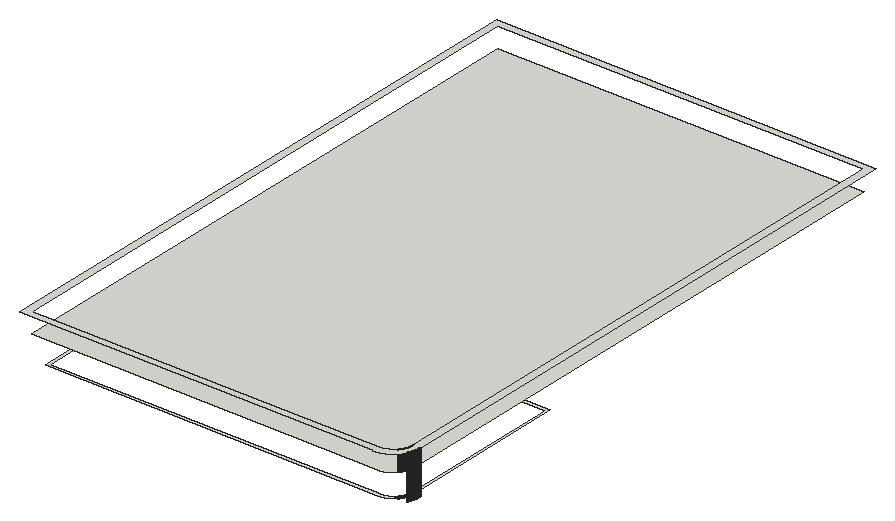
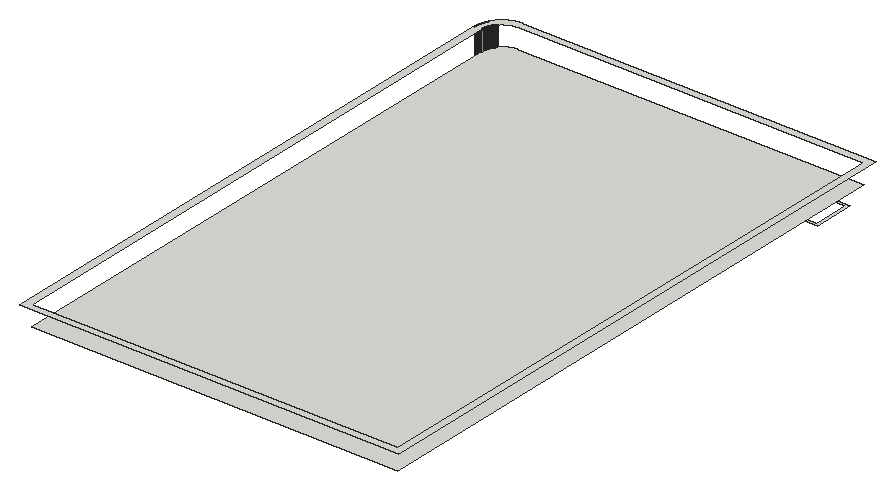
# SketchUp Ruby script. Lengths in inches.
U = 1.inch
M = Sketchup.active_model
def pt(a) = Geom::Point3d.new(a.map { |v| v * U })
def face(e, loops, mat)
  f = e.add_face(loops[0].map { |a| pt(a) })
  loops[1..].each { |l| e.add_face(l.map { |a| pt(a) }).erase! }
  f.material = f.back_material = mat if mat
  f
end
# faces: each face lists its corners as indices into pts; further lists are holes
def faces(e, pts, list, mat = nil) = list.each { |f| face(e, (f[0].is_a?(Array) ? f : [f]).map { |l| l.map { |i| pts[i] } }, mat) }
# xy, xz, yz: faces in a plane at the given z, y or x. An outline is a flat list of corners, or four numbers for a rectangle; further outlines are holes
def ring(l) = l.size == 4 ? [[l[0], l[1]], [l[2], l[1]], [l[2], l[3]], [l[0], l[3]]] : l.each_slice(2).to_a
def flat(e, list, mat, &to3) = list.each { |f| face(e, (f[0].is_a?(Array) ? f : [f]).map { |l| ring(l).map { |u, v| to3.(u, v) } }, mat) }
def xy(e, z, list, mat = nil) = flat(e, list, mat) { |x, y| [x, y, z] }
def xz(e, y, list, mat = nil) = flat(e, list, mat) { |x, z| [x, y, z] }
def yz(e, x, list, mat = nil) = flat(e, list, mat) { |y, z| [x, y, z] }
def lines(e, pts, list) = list.each { |a, b| e.add_line(pt(pts[a]), pt(pts[b])) }
# prism: a flat outline (further loops are holes) pulled along v
def prism(e, loops, v, mat = nil)
  f = face(e, loops, mat); d = Geom::Vector3d.new(v.map { |x| x * U })
  f.pushpull(f.normal.samedirection?(d) ? d.length : -d.length)
end
def box(e, o, s, mat = nil) = prism(e, [[o, [o[0] + s[0], o[1], o[2]], [o[0] + s[0], o[1] + s[1], o[2]], [o[0], o[1] + s[1], o[2]]]], [0, 0, s[2]], mat)
def at(x, y, z, deg = 0) = Geom::Transformation.translation(pt([x, y, z])) * Geom::Transformation.rotation(ORIGIN, Z_AXIS, deg.degrees)
def axes(o, x, y, z) = Geom::Transformation.new([*x, 0, *y, 0, *z, 0, *pt(o).to_a, 1])
def part(name) = M.definitions.add(name)
# library, detail: a bought-in or finely detailed component or shape, given as its bounding box
def library(name, o, s) = part(name).tap { |d| box(d.entities, o, s) }
def detail(e, o, s) = box(e.add_group.entities, o, s)
def put(e, d, t, mat = nil) = e.add_instance(d, t).tap { |i| i.material = mat if mat }
def group(e, t, mat = nil) = e.add_group.tap { |g| g.transformation = t; g.material = mat if mat }.entities
root = M.entities
xy(root,231.5,[[[30,170,30,206,177,206,177,338,342,338,342,187.76,341.99,187.53,341.99,187.29,341.98,187.06,341.96,186.82,341.94,186.59,341.92,186.35,341.9,186.12,341.875,185.88,341.85,185.65,341.8125,185.42,341.78,185.18,341.7,184.72,341.65,184.49,341.61,184.26,341.56,184.03,341.5,183.8,341.45,183.57,341.39,183.34,341.32,183.11,341.26,182.89,341.19,182.66,341.12,182.4375,341.04,182.21,340.97,181.99,340.89,181.77,340.8,181.55,340.72,181.33,340.54,180.89,340.44,180.68,340.35,180.46,340.25,180.25,340.14,180.04,340.04,179.83,339.82,179.41,339.7,179.2,339.59,179,339.35,178.6,339.22,178.39,339.1,178.2,338.97,178,338.83,177.8,338.7,177.61,338.5625,177.42,338.42,177.23,338.28,177.04,338.14,176.86,337.99,176.67,337.84,176.49,337.6875,176.31,337.53,176.13,337.375,175.96,337.22,175.78,337.06,175.61,336.89,175.44,336.73,175.27,336.56,175.11,336.39,174.94,336.22,174.78,336.04,174.625,335.87,174.47,335.69,174.3125,335.51,174.16,335.33,174.01,335.14,173.86,334.96,173.72,334.77,173.58,334.58,173.4375,334.39,173.3,334.2,173.17,334,173.03,333.8,172.9,333.61,172.78,333.4,172.65,333,172.41,332.8,172.3,332.59,172.18,332.17,171.96,331.96,171.86,331.75,171.75,331.54,171.65,331.32,171.56,331.11,171.46,330.67,171.28,330.45,171.2,330.23,171.11,330.01,171.03,329.79,170.96,329.5625,170.88,329.34,170.81,329.11,170.74,328.89,170.68,328.66,170.61,328.43,170.55,328.2,170.5,327.97,170.44,327.74,170.39,327.51,170.35,327.28,170.3,326.82,170.22,326.58,170.1875,326.35,170.15,326.12,170.125,325.88,170.1,325.65,170.08,325.41,170.06,325.18,170.04,324.94,170.02,324.71,170.01,324.47,170.01,324.24,170],[32,172,324.21,172,324.42,172.01,324.63,172.01,325.05,172.03,325.26,172.05,325.46,172.07,325.88,172.11,326.3,172.17,326.5,172.2,326.71,172.23,326.92,172.27,327.12,172.31,327.33,172.35,327.53,172.39,327.74,172.44,327.9375,172.49,328.14,172.55,328.34,172.6,328.94,172.78,329.54,172.99,329.73,173.0625,329.93,173.14,330.12,173.22,330.32,173.3,330.51,173.38,331.08,173.65,331.26,173.74,331.45,173.84,331.63,173.9375,331.82,174.04,332,174.14,332.54,174.47,332.71,174.58,332.89,174.7,333.0625,174.8125,333.23,174.93,333.4,175.06,333.57,175.18,333.74,175.31,333.91,175.43,334.07,175.57,334.39,175.83,334.71,176.11,335.01,176.39,335.16,176.54,335.3125,176.6875,335.46,176.84,335.61,176.99,335.89,177.29,336.17,177.61,336.43,177.93,336.57,178.09,336.69,178.26,336.82,178.43,336.94,178.6,337.07,178.77,337.1875,178.9375,337.3,179.11,337.42,179.29,337.53,179.46,337.86,180,337.96,180.18,338.0625,180.37,338.16,180.55,338.26,180.74,338.35,180.92,338.62,181.49,338.7,181.68,338.78,181.88,338.86,182.07,338.9375,182.27,339.01,182.46,339.22,183.06,339.4,183.66,339.45,183.86,339.51,184.0625,339.56,184.26,339.61,184.47,339.65,184.67,339.69,184.88,339.73,185.08,339.77,185.29,339.8,185.5,339.83,185.7,339.89,186.12,339.93,186.54,339.95,186.74,339.97,186.95,339.99,187.37,339.99,187.58,340,187.79,340,336,179,336,179,204,32,204]]])
xy(root,252,[[18,170,324.24,170,324.47,170.01,324.71,170.01,324.94,170.02,325.18,170.04,325.41,170.06,325.65,170.08,325.88,170.1,326.12,170.125,326.35,170.15,326.58,170.1875,326.82,170.22,327.28,170.3,327.51,170.35,327.74,170.39,327.97,170.44,328.2,170.5,328.43,170.55,328.66,170.61,328.89,170.68,329.11,170.74,329.34,170.81,329.5625,170.88,329.79,170.96,330.01,171.03,330.23,171.11,330.45,171.2,330.67,171.28,331.11,171.46,331.32,171.56,331.54,171.65,331.75,171.75,331.96,171.86,332.17,171.96,332.59,172.18,332.8,172.3,333,172.41,333.4,172.65,333.61,172.78,333.8,172.9,334,173.03,334.2,173.17,334.39,173.3,334.58,173.4375,334.77,173.58,334.96,173.72,335.14,173.86,335.33,174.01,335.51,174.16,335.69,174.3125,335.87,174.47,336.04,174.625,336.22,174.78,336.39,174.94,336.56,175.11,336.73,175.27,336.89,175.44,337.06,175.61,337.22,175.78,337.375,175.96,337.53,176.13,337.6875,176.31,337.84,176.49,337.99,176.67,338.14,176.86,338.28,177.04,338.42,177.23,338.5625,177.42,338.7,177.61,338.83,177.8,338.97,178,339.1,178.2,339.22,178.39,339.35,178.6,339.59,179,339.7,179.2,339.82,179.41,340.04,179.83,340.14,180.04,340.25,180.25,340.35,180.46,340.44,180.68,340.54,180.89,340.72,181.33,340.8,181.55,340.89,181.77,340.97,181.99,341.04,182.21,341.12,182.4375,341.19,182.66,341.26,182.89,341.32,183.11,341.39,183.34,341.45,183.57,341.5,183.8,341.56,184.03,341.61,184.26,341.65,184.49,341.7,184.72,341.78,185.18,341.8125,185.42,341.85,185.65,341.875,185.88,341.9,186.12,341.92,186.35,341.94,186.59,341.96,186.82,341.98,187.06,341.99,187.29,341.99,187.53,342,187.76,342,686,18,686]])
xy(root,270,[[[12,164,324.3125,164,324.63,164.01,324.94,164.02,325.26,164.03,325.88,164.07,326.2,164.1,326.51,164.13,327.44,164.25,327.75,164.3,328.375,164.4,328.68,164.46,328.99,164.52,329.3,164.59,329.6,164.66,329.91,164.74,330.51,164.9,330.82,164.99,331.42,165.17,331.71,165.27,332.31,165.48,332.6,165.59,333.76,166.07,334.05,166.2,334.61,166.48,334.9,166.62,335.17,166.76,335.73,167.06,336,167.22,336.27,167.375,336.54,167.54,336.81,167.7,337.33,168.04,338.11,168.58,338.86,169.15,339.1,169.35,339.35,169.55,339.59,169.75,339.82,169.96,340.06,170.16,340.52,170.59,340.75,170.81,341.19,171.25,341.41,171.48,341.84,171.94,342.04,172.18,342.25,172.41,342.45,172.65,342.65,172.9,342.85,173.14,343.42,173.89,343.96,174.67,344.3,175.19,344.46,175.46,344.625,175.73,344.78,176,344.94,176.27,345.24,176.83,345.38,177.1,345.52,177.39,345.8,177.95,345.93,178.24,346.41,179.4,346.52,179.69,346.73,180.29,346.83,180.58,347.01,181.18,347.1,181.49,347.26,182.09,347.34,182.4,347.41,182.7,347.48,183.01,347.54,183.32,347.6,183.625,347.7,184.25,347.75,184.56,347.87,185.49,347.9,185.8,347.93,186.12,347.97,186.74,347.98,187.06,347.99,187.37,348,187.6875,348,692,12,692],[18,170,18,686,342,686,342,187.76,341.99,187.53,341.99,187.29,341.98,187.06,341.96,186.82,341.94,186.59,341.92,186.35,341.9,186.12,341.875,185.88,341.85,185.65,341.8125,185.42,341.78,185.18,341.7,184.72,341.65,184.49,341.61,184.26,341.56,184.03,341.5,183.8,341.45,183.57,341.39,183.34,341.32,183.11,341.26,182.89,341.19,182.66,341.12,182.4375,341.04,182.21,340.97,181.99,340.89,181.77,340.8,181.55,340.72,181.33,340.54,180.89,340.44,180.68,340.35,180.46,340.25,180.25,340.14,180.04,340.04,179.83,339.82,179.41,339.7,179.2,339.59,179,339.35,178.6,339.22,178.39,339.1,178.2,338.97,178,338.83,177.8,338.7,177.61,338.5625,177.42,338.42,177.23,338.28,177.04,338.14,176.86,337.99,176.67,337.84,176.49,337.6875,176.31,337.53,176.13,337.375,175.96,337.22,175.78,337.06,175.61,336.89,175.44,336.73,175.27,336.56,175.11,336.39,174.94,336.22,174.78,336.04,174.625,335.87,174.47,335.69,174.3125,335.51,174.16,335.33,174.01,335.14,173.86,334.96,173.72,334.77,173.58,334.58,173.4375,334.39,173.3,334.2,173.17,334,173.03,333.8,172.9,333.61,172.78,333.4,172.65,333,172.41,332.8,172.3,332.59,172.18,332.17,171.96,331.96,171.86,331.75,171.75,331.54,171.65,331.32,171.56,331.11,171.46,330.67,171.28,330.45,171.2,330.23,171.11,330.01,171.03,329.79,170.96,329.5625,170.88,329.34,170.81,329.11,170.74,328.89,170.68,328.66,170.61,328.43,170.55,328.2,170.5,327.97,170.44,327.74,170.39,327.51,170.35,327.28,170.3,326.82,170.22,326.58,170.1875,326.35,170.15,326.12,170.125,325.88,170.1,325.65,170.08,325.41,170.06,325.18,170.04,324.94,170.02,324.71,170.01,324.47,170.01,324.24,170]]])
yz(root,339.99,[[187.37,231,187.58,231.5]])
yz(root,341.99,[[187.29,231,187.53,231.5],[187.29,252,187.53,270]])
yz(root,342,[[187.76,231,188,231.5],[187.76,252,188,270]])
yz(root,348,[[187.6875,231,188,270]])
p = [[334.71,176.11,231],[334.86,176.25,231],[334.86,176.25,231.5],[334.71,176.11,231.5],[337.6875,176.31,231],[337.53,176.13,231],
  [337.53,176.13,231.5],[337.6875,176.31,231.5],[335.01,176.39,231],[335.01,176.39,231.5],[337.84,176.49,231],[337.84,176.49,231.5],
  [345.09,176.55,231],[345.09,176.55,270],[344.94,176.27,270],[344.94,176.27,231],[335.16,176.54,231],[335.16,176.54,231.5],
  [335.3125,176.6875,231],[335.3125,176.6875,231.5],[337.99,176.67,231],[337.99,176.67,231.5],[345.24,176.83,231],[345.24,176.83,270],
  [335.46,176.84,231],[335.46,176.84,231.5],[338.14,176.86,231],[338.14,176.86,231.5],[335.61,176.99,231],[335.61,176.99,231.5],
  [345.38,177.1,231],[345.38,177.1,270],[338.28,177.04,231],[338.28,177.04,231.5],[335.75,177.14,231],[335.75,177.14,231.5],
  [338.42,177.23,231],[338.42,177.23,231.5],[335.89,177.29,231],[335.89,177.29,231.5],[345.52,177.39,231],[345.52,177.39,270],
  [338.5625,177.42,231],[338.5625,177.42,231.5],[336.03,177.45,231],[336.03,177.45,231.5],[338.7,177.61,231],[338.7,177.61,231.5],
  [345.66,177.67,231],[345.66,177.67,270],[336.17,177.61,231],[336.17,177.61,231.5],[336.3,177.77,231],[336.3,177.77,231.5],
  [338.83,177.8,231],[338.83,177.8,231.5],[345.8,177.95,231],[345.8,177.95,270],[336.43,177.93,231],[336.43,177.93,231.5],
  [338.97,178,231],[338.97,178,231.5],[336.57,178.09,231],[336.57,178.09,231.5],[339.1,178.2,231],[339.1,178.2,231.5],
  [345.93,178.24,231],[345.93,178.24,270],[336.69,178.26,231],[336.69,178.26,231.5],[339.22,178.39,231],[339.22,178.39,231.5],
  [346.05,178.53,231],[346.05,178.53,270],[336.82,178.43,231],[336.82,178.43,231.5],[336.94,178.6,231],[336.94,178.6,231.5],
  [339.35,178.6,231],[339.35,178.6,231.5],[346.17,178.82,231],[346.17,178.82,270],[337.07,178.77,231],[337.07,178.77,231.5],
  [339.47,178.8,231],[339.47,178.8,231.5],[337.1875,178.9375,231],[337.1875,178.9375,231.5],[339.59,179,231],[339.59,179,231.5],
  [346.29,179.11,231],[346.29,179.11,270],[337.3,179.11,231],[337.3,179.11,231.5],[339.7,179.2,231],[339.7,179.2,231.5],
  [337.42,179.29,231],[337.42,179.29,231.5],[346.41,179.4,231],[346.41,179.4,270],[339.82,179.41,231],[339.82,179.41,231.5],
  [337.53,179.46,231],[337.53,179.46,231.5],[339.93,179.62,231],[339.93,179.62,231.5],[346.52,179.69,231],[346.52,179.69,270],
  [337.64,179.64,231],[337.64,179.64,231.5],[337.75,179.82,231],[337.75,179.82,231.5],[340.04,179.83,231],[340.04,179.83,231.5],
  [346.625,179.99,231],[346.625,179.99,270],[337.86,180,231],[337.86,180,231.5],[340.14,180.04,231],[340.14,180.04,231.5],
  [337.96,180.18,231],[337.96,180.18,231.5],[340.25,180.25,231],[340.25,180.25,231.5],[346.73,180.29,231],[346.73,180.29,270],
  [338.0625,180.37,231],[338.0625,180.37,231.5],[340.35,180.46,231],[340.35,180.46,231.5],[346.83,180.58,231],[346.83,180.58,270],
  [338.16,180.55,231],[338.16,180.55,231.5],[340.44,180.68,231],[340.44,180.68,231.5],[338.26,180.74,231],[338.26,180.74,231.5],
  [346.92,180.88,231],[346.92,180.88,270],[338.35,180.92,231],[338.35,180.92,231.5],[340.54,180.89,231],[340.54,180.89,231.5],
  [338.44,181.11,231],[338.44,181.11,231.5],[340.63,181.11,231],[340.63,181.11,231.5],[347.01,181.18,231],[347.01,181.18,270],
  [338.53,181.3,231],[338.53,181.3,231.5],[340.72,181.33,231],[340.72,181.33,231.5],[347.1,181.49,231],[347.1,181.49,270],
  [338.62,181.49,231],[338.62,181.49,231.5],[340.8,181.55,231],[340.8,181.55,231.5],[338.7,181.68,231],[338.7,181.68,231.5],
  [340.89,181.77,231],[340.89,181.77,231.5],[347.18,181.79,231],[347.18,181.79,270],[338.78,181.88,231],[338.78,181.88,231.5],
  [340.97,181.99,231],[340.97,181.99,231.5],[347.26,182.09,231],[347.26,182.09,270],[338.86,182.07,231],[338.86,182.07,231.5],
  [341.04,182.21,231],[341.04,182.21,231.5],[338.9375,182.27,231],[338.9375,182.27,231.5],[347.34,182.4,231],[347.34,182.4,270],
  [341.12,182.4375,231],[341.12,182.4375,231.5],[339.01,182.46,231],[339.01,182.46,231.5],[341.19,182.66,231],[341.19,182.66,231.5],
  [347.41,182.7,231],[347.41,182.7,270],[339.08,182.66,231],[339.08,182.66,231.5],[339.15,182.86,231],[339.15,182.86,231.5],
  [341.26,182.89,231],[341.26,182.89,231.5],[347.48,183.01,231],[347.48,183.01,270],[339.22,183.06,231],[339.22,183.06,231.5],
  [341.32,183.11,231],[341.32,183.11,231.5],[347.54,183.32,231],[347.54,183.32,270],[339.28,183.26,231],[339.28,183.26,231.5],
  [341.39,183.34,231],[341.39,183.34,231.5],[339.34,183.46,231],[339.34,183.46,231.5],[341.45,183.57,231],[341.45,183.57,231.5],
  [347.6,183.625,231],[347.6,183.625,270],[339.4,183.66,231],[339.4,183.66,231.5],[341.5,183.8,231],[341.5,183.8,231.5],
  [347.65,183.9375,231],[347.65,183.9375,270],[339.45,183.86,231],[339.45,183.86,231.5],[341.56,184.03,231],[341.56,184.03,231.5],
  [339.51,184.0625,231],[339.51,184.0625,231.5],[347.7,184.25,231],[347.7,184.25,270],[341.61,184.26,231],[341.61,184.26,231.5],
  [339.56,184.26,231],[339.56,184.26,231.5],[347.75,184.56,231],[347.75,184.56,270],[339.61,184.47,231],[339.61,184.47,231.5],
  [341.65,184.49,231],[341.65,184.49,231.5],[339.65,184.67,231],[339.65,184.67,231.5],[341.7,184.72,231],[341.7,184.72,231.5],
  [347.79,184.87,231],[347.79,184.87,270],[339.69,184.88,231],[339.69,184.88,231.5],[341.74,184.95,231],[341.74,184.95,231.5],
  [339.73,185.08,231],[339.73,185.08,231.5],[347.83,185.18,231],[347.83,185.18,270],[341.78,185.18,231],[341.78,185.18,231.5],
  [339.77,185.29,231],[339.77,185.29,231.5],[341.8125,185.42,231],[341.8125,185.42,231.5],[347.87,185.49,231],[347.87,185.49,270],
  [339.8,185.5,231],[339.8,185.5,231.5],[341.85,185.65,231],[341.85,185.65,231.5],[339.83,185.7,231],[339.83,185.7,231.5],
  [347.9,185.8,231],[347.9,185.8,270],[339.86,185.91,231],[339.86,185.91,231.5],[341.875,185.88,231],[341.875,185.88,231.5],
  [347.93,186.12,231],[347.93,186.12,270],[339.89,186.12,231],[339.89,186.12,231.5],[341.9,186.12,231],[341.9,186.12,231.5],
  [339.91,186.33,231],[339.91,186.33,231.5],[341.92,186.35,231],[341.92,186.35,231.5],[347.95,186.43,231],[347.95,186.43,270],
  [339.93,186.54,231],[339.93,186.54,231.5],[341.94,186.59,231],[341.94,186.59,231.5],[347.97,186.74,231],[347.97,186.74,270],
  [339.95,186.74,231],[339.95,186.74,231.5],[341.96,186.82,231],[341.96,186.82,231.5],[339.97,186.95,231],[339.97,186.95,231.5],
  [347.98,187.06,231],[347.98,187.06,270],[341.98,187.06,231],[341.98,187.06,231.5],[339.98,187.16,231],[339.98,187.16,231.5],
  [341.99,187.29,231],[341.99,187.29,231.5],[347.99,187.37,231],[347.99,187.37,270],[339.99,187.37,231],[339.99,187.37,231.5],
  [348,187.6875,231],[348,187.6875,270],[342,187.76,231],[341.99,187.53,231],[341.99,187.53,231.5],[342,187.76,231.5],
  [339.99,187.58,231],[340,187.79,231],[340,187.79,231.5],[339.99,187.58,231.5],[337.6875,176.31,252],[337.53,176.13,252],
  [337.53,176.13,270],[337.6875,176.31,270],[337.84,176.49,252],[337.84,176.49,270],[337.99,176.67,252],[337.99,176.67,270],
  [338.14,176.86,252],[338.14,176.86,270],[338.28,177.04,252],[338.28,177.04,270],[338.42,177.23,252],[338.42,177.23,270],
  [338.5625,177.42,252],[338.5625,177.42,270],[338.7,177.61,252],[338.7,177.61,270],[338.83,177.8,252],[338.83,177.8,270],
  [338.97,178,252],[338.97,178,270],[339.1,178.2,252],[339.1,178.2,270],[339.22,178.39,252],[339.22,178.39,270],
  [339.35,178.6,252],[339.35,178.6,270],[339.47,178.8,252],[339.47,178.8,270],[339.59,179,252],[339.59,179,270],
  [339.7,179.2,252],[339.7,179.2,270],[339.82,179.41,252],[339.82,179.41,270],[339.93,179.62,252],[339.93,179.62,270],
  [340.04,179.83,252],[340.04,179.83,270],[340.14,180.04,252],[340.14,180.04,270],[340.25,180.25,252],[340.25,180.25,270],
  [340.35,180.46,252],[340.35,180.46,270],[340.44,180.68,252],[340.44,180.68,270],[340.54,180.89,252],[340.54,180.89,270],
  [340.63,181.11,252],[340.63,181.11,270],[340.72,181.33,252],[340.72,181.33,270],[340.8,181.55,252],[340.8,181.55,270],
  [340.89,181.77,252],[340.89,181.77,270],[340.97,181.99,252],[340.97,181.99,270],[341.04,182.21,252],[341.04,182.21,270],
  [341.12,182.4375,252],[341.12,182.4375,270],[341.19,182.66,252],[341.19,182.66,270],[341.26,182.89,252],[341.26,182.89,270],
  [341.32,183.11,252],[341.32,183.11,270],[341.39,183.34,252],[341.39,183.34,270],[341.45,183.57,252],[341.45,183.57,270],
  [341.5,183.8,252],[341.5,183.8,270],[341.56,184.03,252],[341.56,184.03,270],[341.61,184.26,252],[341.61,184.26,270],
  [341.65,184.49,252],[341.65,184.49,270],[341.7,184.72,252],[341.7,184.72,270],[341.74,184.95,252],[341.74,184.95,270],
  [341.78,185.18,252],[341.78,185.18,270],[341.8125,185.42,252],[341.8125,185.42,270],[341.85,185.65,252],[341.85,185.65,270],
  [341.875,185.88,252],[341.875,185.88,270],[341.9,186.12,252],[341.9,186.12,270],[341.92,186.35,252],[341.92,186.35,270],
  [341.94,186.59,252],[341.94,186.59,270],[341.96,186.82,252],[341.96,186.82,270],[341.98,187.06,252],[341.98,187.06,270],
  [341.99,187.29,252],[341.99,187.29,270],[342,187.76,252],[341.99,187.53,252],[341.99,187.53,270],[342,187.76,270]]
faces(root,p,[[0,1,2,3],[4,5,6,7],[1,8,9,2],[10,4,7,11],[12,13,14,15],[8,16,17,9],[16,18,19,17],[20,10,11,21],
  [22,23,13,12],[18,24,25,19],[26,20,21,27],[24,28,29,25],[30,31,23,22],[32,26,27,33],[28,34,35,29],[36,32,33,37],
  [34,38,39,35],[40,41,31,30],[42,36,37,43],[38,44,45,39],[46,42,43,47],[48,49,41,40],[44,50,51,45],[50,52,53,51],
  [54,46,47,55],[56,57,49,48],[52,58,59,53],[60,54,55,61],[58,62,63,59],[64,60,61,65],[66,67,57,56],[62,68,69,63],
  [70,64,65,71],[72,73,67,66],[68,74,75,69],[74,76,77,75],[78,70,71,79],[80,81,73,72],[76,82,83,77],[84,78,79,85],
  [82,86,87,83],[88,84,85,89],[90,91,81,80],[86,92,93,87],[94,88,89,95],[92,96,97,93],[98,99,91,90],[100,94,95,101],
  [96,102,103,97],[104,100,101,105],[106,107,99,98],[102,108,109,103],[108,110,111,109],[112,104,105,113],[114,115,107,106],[110,116,117,111],
  [118,112,113,119],[116,120,121,117],[122,118,119,123],[124,125,115,114],[120,126,127,121],[128,122,123,129],[130,131,125,124],[126,132,133,127],
  [134,128,129,135],[132,136,137,133],[138,139,131,130],[136,140,141,137],[142,134,135,143],[140,144,145,141],[146,142,143,147],[148,149,139,138],
  [144,150,151,145],[152,146,147,153],[154,155,149,148],[150,156,157,151],[158,152,153,159],[156,160,161,157],[162,158,159,163],[164,165,155,154],
  [160,166,167,161],[168,162,163,169],[170,171,165,164],[166,172,173,167],[174,168,169,175],[172,176,177,173],[178,179,171,170],[180,174,175,181],
  [176,182,183,177],[184,180,181,185],[186,187,179,178],[182,188,189,183],[188,190,191,189],[192,184,185,193],[194,195,187,186],[190,196,197,191],
  [198,192,193,199],[200,201,195,194],[196,202,203,197],[204,198,199,205],[202,206,207,203],[208,204,205,209],[210,211,201,200],[206,212,213,207],
  [214,208,209,215],[216,217,211,210],[212,218,219,213],[220,214,215,221],[218,222,223,219],[224,225,217,216],[226,220,221,227],[222,228,229,223],
  [230,231,225,224],[228,232,233,229],[234,226,227,235],[232,236,237,233],[238,234,235,239],[240,241,231,230],[236,242,243,237],[244,238,239,245],
  [242,246,247,243],[248,249,241,240],[250,244,245,251],[246,252,253,247],[254,250,251,255],[256,257,249,248],[252,258,259,253],[260,254,255,261],
  [258,262,263,259],[264,265,257,256],[262,266,267,263],[268,260,261,269],[270,271,265,264],[266,272,273,267],[274,268,269,275],[272,276,277,273],
  [278,274,275,279],[280,281,271,270],[276,282,283,277],[284,278,279,285],[286,287,281,280],[282,288,289,283],[290,284,285,291],[288,292,293,289],
  [294,295,287,286],[296,290,291,297],[292,298,299,293],[300,296,297,301],[302,303,295,294],[298,304,305,299],[306,307,303,302],[308,309,310,311],
  [312,313,314,315],[316,317,318,319],[320,316,319,321],[322,320,321,323],[324,322,323,325],[326,324,325,327],[328,326,327,329],[330,328,329,331],
  [332,330,331,333],[334,332,333,335],[336,334,335,337],[338,336,337,339],[340,338,339,341],[342,340,341,343],[344,342,343,345],[346,344,345,347],
  [348,346,347,349],[350,348,349,351],[352,350,351,353],[354,352,353,355],[356,354,355,357],[358,356,357,359],[360,358,359,361],[362,360,361,363],
  [364,362,363,365],[366,364,365,367],[368,366,367,369],[370,368,369,371],[372,370,371,373],[374,372,373,375],[376,374,375,377],[378,376,377,379],
  [380,378,379,381],[382,380,381,383],[384,382,383,385],[386,384,385,387],[388,386,387,389],[390,388,389,391],[392,390,391,393],[394,392,393,395],
  [396,394,395,397],[398,396,397,399],[400,398,399,401],[402,400,401,403],[404,402,403,405],[406,404,405,407],[408,406,407,409],[410,408,409,411],
  [412,410,411,413],[414,412,413,415],[416,414,415,417],[418,416,417,419],[420,418,419,421],[422,423,424,425]])
